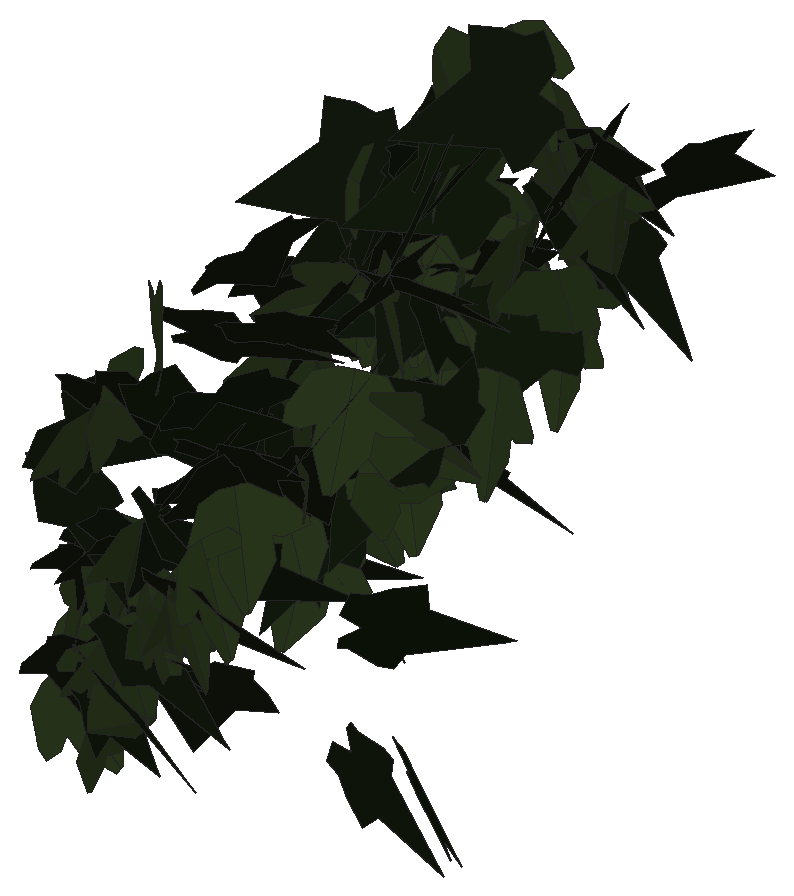
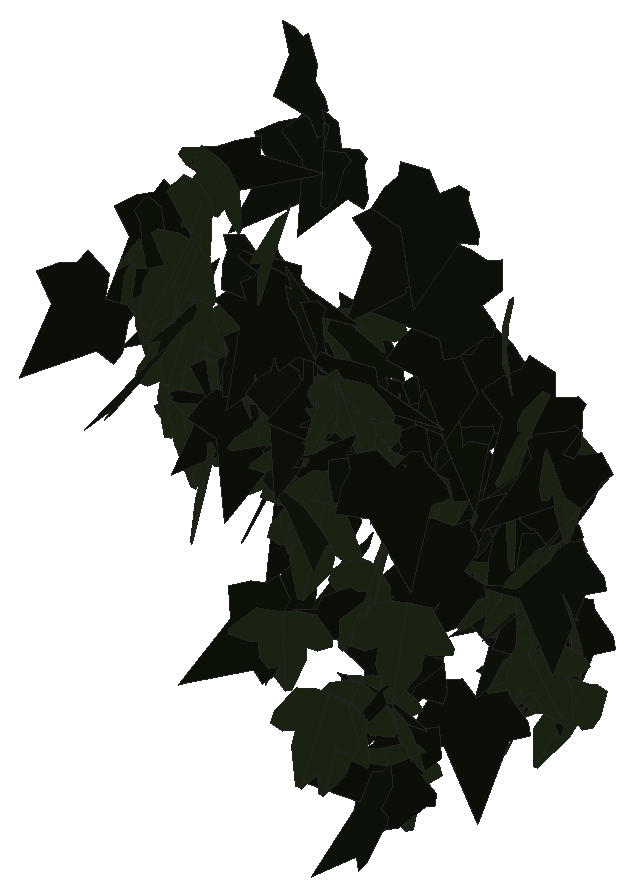
# SketchUp Ruby script. Lengths in inches.
U = 1.inch
M = Sketchup.active_model
def pt(a) = Geom::Point3d.new(a.map { |v| v * U })
def face(e, loops, mat)
  f = e.add_face(loops[0].map { |a| pt(a) })
  loops[1..].each { |l| e.add_face(l.map { |a| pt(a) }).erase! }
  f.material = f.back_material = mat if mat
  f
end
# faces: each face lists its corners as indices into pts; further lists are holes
def faces(e, pts, list, mat = nil) = list.each { |f| face(e, (f[0].is_a?(Array) ? f : [f]).map { |l| l.map { |i| pts[i] } }, mat) }
# xy, xz, yz: faces in a plane at the given z, y or x. An outline is a flat list of corners, or four numbers for a rectangle; further outlines are holes
def ring(l) = l.size == 4 ? [[l[0], l[1]], [l[2], l[1]], [l[2], l[3]], [l[0], l[3]]] : l.each_slice(2).to_a
def flat(e, list, mat, &to3) = list.each { |f| face(e, (f[0].is_a?(Array) ? f : [f]).map { |l| ring(l).map { |u, v| to3.(u, v) } }, mat) }
def xy(e, z, list, mat = nil) = flat(e, list, mat) { |x, y| [x, y, z] }
def xz(e, y, list, mat = nil) = flat(e, list, mat) { |x, z| [x, y, z] }
def yz(e, x, list, mat = nil) = flat(e, list, mat) { |y, z| [x, y, z] }
def lines(e, pts, list) = list.each { |a, b| e.add_line(pt(pts[a]), pt(pts[b])) }
# prism: a flat outline (further loops are holes) pulled along v
def prism(e, loops, v, mat = nil)
  f = face(e, loops, mat); d = Geom::Vector3d.new(v.map { |x| x * U })
  f.pushpull(f.normal.samedirection?(d) ? d.length : -d.length)
end
def box(e, o, s, mat = nil) = prism(e, [[o, [o[0] + s[0], o[1], o[2]], [o[0] + s[0], o[1] + s[1], o[2]], [o[0], o[1] + s[1], o[2]]]], [0, 0, s[2]], mat)
def at(x, y, z, deg = 0) = Geom::Transformation.translation(pt([x, y, z])) * Geom::Transformation.rotation(ORIGIN, Z_AXIS, deg.degrees)
def axes(o, x, y, z) = Geom::Transformation.new([*x, 0, *y, 0, *z, 0, *pt(o).to_a, 1])
def part(name) = M.definitions.add(name)
# library, detail: a bought-in or finely detailed component or shape, given as its bounding box
def library(name, o, s) = part(name).tap { |d| box(d.entities, o, s) }
def detail(e, o, s) = box(e.add_group.entities, o, s)
def put(e, d, t, mat = nil) = e.add_instance(d, t).tap { |i| i.material = mat if mat }
def group(e, t, mat = nil) = e.add_group.tap { |g| g.transformation = t; g.material = mat if mat }.entities
root = M.entities
M.materials.add("efeu1").color = [18, 25, 13]
M.materials.add("efeu2").color = [43, 57, 29]
c1 = part("ivyleaf_9")
p = [[1.54,2.16,1.25],[1.36,2.04,1.19],[-0.21,0.99,0.68],[-0.71,1.11,0.82],[-0.85,0.86,0.67],[-0.8,0.17,0.21],
  [-0.9,-0.01,0.1],[-0.67,-0.16,-0.02],[-0.08,-0.08,-0.05],[-0.03,-0.6,-0.4],[0.65,-0.88,-0.66],[0.83,-0.6,-0.49],
  [1.29,-0.42,-0.43],[1.8125,-0.07,-0.26],[1.21,0.44,0.15]]
faces(c1.entities,p,[[0,1,2,3,4,5,6,7,8,9,10,11,12,13,14]],"efeu1")
c2 = part("ivyleaf_10")
p = [[0,0.5,-0.03],[-0.0625,2.02,-0.43],[-0.19,2.01,-0.46],[-0.54,1.05,-0.29],[-0.52,0.625,-0.18],[-0.83,0.76,-0.28],
  [-1.16,0.64,-0.33],[-1.15,0.33,-0.24],[-0.77,-0.39,0.02],[-0.3,-0.51,0.16],[0.04,-0.48,0.23],[-0.02,2.01,-0.4375],
  [-0.06,2.01,-0.43],[0.04,-0.49,0.23],[0.67,-0.49,0.14],[1.38,0.36,-0.2],[1.375,0.51,-0.24],[0.81,0.65,-0.19],
  [0.62,0.59,-0.15],[0.6,1.09,-0.28],[0.5,1.23,-0.31]]
faces(c2.entities,p,[[0,1,2,3,4,5,6,7,8,9,10],[11,12,0,13,14,15,16,17,18,19,20]],"efeu2")
put(root,c1,axes([34.97,224.375,226.84],[0.18635,-0.03833,0.46239],[0.45579,-0.07806,-0.19016],[0.08677,0.49238,0.00585]))
put(root,c1,axes([33.65,224.56,225.77],[0.23627,-0.43906,-0.03737],[0.01842,0.05221,-0.49693],[0.44027,0.23344,0.04084]))
put(root,c1,axes([38.15,224.08,230.05],[0.09512,0.13668,0.47145],[0.01693,0.47903,-0.14229],[-0.49058,0.04304,0.08651]))
put(root,c2,axes([34.26,224.52,224.04],[-0.01331,-0.49982,-0.00062],[0.00269,0.00055,-0.49999],[0.49982,-0.01332,0.00267]))
put(root,c1,axes([36.35,224.14,228.54],[0.41156,0.27456,0.07234],[-0.00014,0.12759,-0.48345],[-0.28393,0.39792,0.1051]))
put(root,c2,axes([34.46,224.55,225.35],[0.05486,-0.49669,0.01713],[0.00671,-0.01649,-0.49968],[0.49694,0.05505,0.00486]))
put(root,c2,axes([33.9,224.47,226.4],[-0.0166,-0.49344,-0.07903],[0.00415,0.07893,-0.49371],[0.49971,-0.01705,0.00148]))
put(root,c2,axes([35.52,224.38,225.48],[0.07164,0.49096,0.06186],[0.00259,0.06213,-0.49612],[-0.49483,0.07141,0.00636]))
put(root,c1,axes([34.09,224.57,223.64],[0.35748,-0.3082,0.165],[0.14154,-0.0882,-0.47137],[0.31965,0.38372,0.02419]))
put(root,c1,axes([34.47,224.5,224.3125],[0.33175,-0.37154,-0.04357],[0.07631,0.12422,-0.47827],[0.36622,0.31069,0.13913]))
put(root,c1,axes([35.02,224.45,224.89],[0.39681,-0.14655,0.26658],[0.27236,-0.02402,-0.41862],[0.1355,0.47744,0.06077]))
put(root,c2,axes([35.15,224.43,225.04],[0.05746,-0.46499,-0.17458],[0.00556,0.17634,-0.46784],[0.49666,0.05183,0.02544]))
put(root,c2,axes([35.17,224.42,224.99],[-0.14905,0.47635,0.02964],[-0.00164,0.03054,-0.49906],[-0.47726,-0.14887,-0.00754]))
put(root,c1,axes([34.05,224.36,224.1],[0.19728,0.42233,-0.18089],[-0.08261,-0.16105,-0.46609],[-0.45195,0.21379,0.00624]))
put(root,c1,axes([36.08,224.24,229.21],[0.12055,0.48298,0.04692],[-0.00865,0.05048,-0.49737],[-0.48517,0.1191,0.02053]))
put(root,c1,axes([35.36,224.36,228.01],[0.38179,-0.06892,0.31542],[0.32286,0.08327,-0.3726],[-0.00117,0.48818,0.10809]))
put(root,c1,axes([34.23,224.31,227.04],[0.45045,0.21425,-0.03449],[-0.04369,0.0117,-0.49795],[-0.21257,0.45162,0.02926]))
put(root,c1,axes([37.56,224.28,225.56],[0.33918,0.12741,0.34457],[0.32373,0.11804,-0.36231],[-0.17367,0.46886,-0.00241]))
put(root,c1,axes([37.66,224.1875,229.3],[0.10481,0.41722,0.25484],[0.01741,0.25728,-0.42838],[-0.48858,0.09866,0.0394]))
put(root,c2,axes([34.25,224.24,223.32],[0.01123,-0.18738,-0.46343],[0.07848,0.45846,-0.18346],[0.49368,-0.06862,0.0397]))
put(root,c2,axes([33.71,224.64,224.45],[0.33781,-0.36812,-0.01926],[0.01049,0.03571,-0.49861],[0.36847,0.33647,0.03185]))
put(root,c2,axes([34.96,224.27,227.7],[-0.0367,0.04037,-0.49701],[-0.20273,0.4541,0.05186],[0.45558,0.20533,-0.01696]))
put(root,c1,axes([34.48,224.54,225.44],[0.19978,0.33296,-0.315],[-0.16852,-0.2662,-0.38825],[-0.42625,0.2613,0.00586]))
put(root,c2,axes([34.75,224.52,224.67],[-0.11062,0.487,0.02429],[-0.00816,0.02306,-0.4994],[-0.48754,-0.11089,0.00284]))
put(root,c2,axes([34.3,224.57,224.19],[-0.35728,-0.33193,-0.11033],[0.11029,0.04276,-0.48581],[0.33194,-0.37148,0.04266]))
put(root,c1,axes([34.68,224.66,225.64],[0.37166,-0.33425,-0.01217],[-0.01358,0.0031,-0.49981],[0.33419,0.37184,-0.00678]))
put(root,c1,axes([35.62,224.39,227.39],[0.23033,0.43977,-0.05959],[-0.02845,-0.05237,-0.49644],[-0.44287,0.23208,0.0009]))
put(root,c1,axes([35.55,224.43,226.69],[-0.08089,0.4934,0.00325],[-0.00346,0.00273,-0.49998],[-0.4934,-0.08091,0.00297]))
put(root,c1,axes([34.31,224.57,225.24],[-0.0586,0.4589,-0.18969],[-0.01655,-0.1927,-0.46108],[-0.49628,-0.04776,0.03778]))
put(root,c1,axes([33.99,224.54,223.71],[0.285,-0.246,-0.32903],[-0.24122,0.22395,-0.37638],[0.33255,0.37327,0.00897]))
put(root,c2,axes([34.86,224.47,224.7],[-0.11811,-0.34206,-0.34503],[0.13572,0.31771,-0.36144],[0.46651,-0.17903,0.0178]))
put(root,c2,axes([34.27,224.43,226.83],[0.01596,-0.28426,-0.41103],[0.11959,0.40146,-0.273],[0.48522,-0.0896,0.0808]))
put(root,c1,axes([35.58,224.45,226.71],[0.41641,0.25774,-0.10087],[-0.13834,0.03599,-0.47913],[-0.23972,0.42694,0.10129]))
put(root,c1,axes([37.11,224.65,223.79],[0.37319,-0.29128,-0.16089],[-0.08169,0.15415,-0.46858],[0.32258,0.37602,0.06747]))
put(root,c1,axes([35.2,224.42,226.07],[0.27285,0.01724,0.41864],[0.32924,0.30016,-0.22695],[-0.25914,0.39951,0.15244]))
put(root,c1,axes([37.75,224.47,229.36],[0.48326,0.12752,0.01403],[-0.02325,0.14081,-0.4792],[-0.12616,0.4625,0.14203]))
put(root,c1,axes([33.78,224.42,226.45],[0.05481,0.0184,-0.49665],[-0.08435,0.49275,0.00894],[0.48978,0.0828,0.05711]))
put(root,c2,axes([34.07,224.62,225],[-0.03441,0.48265,0.12597],[0.00493,0.1266,-0.48368],[-0.49879,-0.03205,-0.01347]))
put(root,c1,axes([34,224.6,225.05],[0.15996,0.45543,-0.13037],[-0.14225,-0.08507,-0.47173],[-0.45186,0.188,0.10235]))
put(root,c2,axes([35.54,224.79,225.89],[0.25289,0.43,0.03383],[0.01791,0.02871,-0.49885],[-0.43096,0.25352,-0.00088]))
put(root,c1,axes([34.22,224.55,223.96],[0.42873,0.25704,-0.01107],[-0.08616,0.12317,-0.47687],[-0.24243,0.4108,0.14991]))
put(root,c2,axes([33.5625,224.66,223.26],[0.14624,0.40594,0.25265],[0.06465,0.24499,-0.43105],[-0.47375,0.15874,0.01916]))
put(root,c2,axes([36.78,224.95,227.55],[0.42652,0.25364,-0.06118],[-0.05138,-0.0333,-0.49624],[-0.25581,0.4296,-0.00235]))
put(root,c1,axes([37.66,224.84,223.68],[0.37525,-0.06365,-0.32425],[-0.312,0.09333,-0.3794],[0.10882,0.48707,0.03033]))
put(root,c1,axes([36.74,224.74,227.32],[-0.07383,0.45234,0.19984],[-0.04646,0.19481,-0.45814],[-0.49233,-0.08622,0.01327]))
put(root,c2,axes([34.01,225.05,224.01],[-0.06553,0.4942,-0.03832],[0.02094,-0.03586,-0.49827],[-0.49525,-0.0669,-0.016]))
put(root,c2,axes([33.75,225.21,223.9],[0.36328,0.29795,-0.17103],[-0.14426,-0.09361,-0.4695],[-0.31179,0.39046,0.01795]))
put(root,c1,axes([36,224.92,226.5625],[0.32823,0.36541,-0.09349],[-0.09347,-0.04126,-0.48945],[-0.36541,0.33878,0.04122]))
put(root,c2,axes([37.13,225.11,227.23],[0.14676,-0.04549,0.47581],[0.43833,0.21128,-0.115],[-0.19059,0.45088,0.1019]))
put(root,c2,axes([36.1,225.09,226.32],[-0.01835,0.05933,-0.49613],[-0.18096,0.46197,0.06194],[0.46574,0.18183,0.00452]))
put(root,c1,axes([37.7,225.25,227.21],[-0.12889,0.31143,0.36933],[-0.26609,0.27327,-0.32329],[-0.40322,-0.27988,0.09529]))
put(root,c1,axes([34.93,225.24,224.82],[0.39504,0.11042,0.28592],[0.26654,0.1065,-0.40941],[-0.15132,0.47588,0.02528]))
put(root,c2,axes([36.79,225.4,226.52],[0.02656,-0.16915,-0.46977],[0.28001,0.39454,-0.12623],[0.41339,-0.25637,0.11569]))
put(root,c1,axes([34.36,225.625,223.33],[0.27028,0.33175,-0.25862],[-0.19766,-0.17119,-0.42617],[-0.37132,0.33261,0.03861]))
put(root,c2,axes([37.81,225.88,227.47],[0.48557,-0.08914,0.07925],[0.0791,-0.00798,-0.49364],[0.08927,0.49193,0.00635]))
put(root,c2,axes([36.29,226.39,226.1],[0.40949,0.27125,0.0935],[0.07274,0.05946,-0.49109],[-0.27754,0.4158,0.00923]))
put(root,c1,axes([37.48,226.91,230.26],[-0.31936,-0.17974,0.34015],[-0.29297,-0.17291,-0.36643],[0.24936,-0.43335,0.00513]))
put(root,c1,axes([36.78,226.96,229.04],[-0.43607,-0.04937,0.2396],[-0.24019,-0.00648,-0.43848],[0.0464,-0.49751,-0.01807]))
put(root,c2,axes([35.59,226.97,227.51],[-0.19592,0.22951,-0.39867],[0.23812,-0.32016,-0.30133],[-0.39359,-0.30793,0.01615]))
put(root,c2,axes([34.5,226.79,224.76],[0.30737,0.37801,0.11238],[0.06557,0.09151,-0.48716],[-0.38887,0.31422,0.00668]))
put(root,c2,axes([35.13,227.04,227.15],[0.13266,0.16472,-0.45307],[-0.45772,-0.10446,-0.172],[-0.15132,0.46038,0.12308]))
put(root,c1,axes([35.14,226.96,227.28],[-0.19985,0.39523,-0.23207],[0.0831,-0.21772,-0.44237],[-0.45073,-0.21539,0.02134]))
put(root,c1,axes([35.9,226.6875,226.38],[0.32872,0.37577,0.02711],[0.01844,0.01989,-0.49926],[-0.3763,0.32924,-0.00078]))
put(root,c1,axes([35.95,227.17,229.1875],[-0.38006,0.16701,-0.27868],[0.24981,-0.124,-0.41499],[-0.20773,-0.45468,0.01081]))
put(root,c1,axes([34.5,226.73,224.53],[0.24677,0.42688,0.08291],[0.03885,0.07331,-0.49307],[-0.43312,0.24979,0.00302]))
put(root,c1,axes([36.76,226.88,229.27],[-0.15033,0.47683,0.00594],[-0.00217,0.00555,-0.49996],[-0.47686,-0.15034,0.0004]))
put(root,c2,axes([37.1,227.25,230.47],[-0.39682,0.05542,-0.29911],[0.24243,-0.23935,-0.36598],[-0.18374,-0.43548,0.16308]))
put(root,c1,axes([35.36,227.22,228.21],[-0.46425,0.18541,0.00945],[-0.01291,-0.00686,-0.49979],[-0.18521,-0.4643,0.01115]))
put(root,c2,axes([35.49,227.34,226.63],[-0.01902,0.44977,-0.21759],[-0.01191,-0.21809,-0.44977],[-0.4995,-0.01193,0.01901]))
put(root,c1,axes([37.95,227.23,229.65],[-0.2531,0.38959,-0.18482],[0.11116,-0.14812,-0.46444],[-0.41664,-0.27619,-0.01163]))
put(root,c2,axes([36.96,227.35,228.26],[0.08534,-0.48994,0.05171],[0.00389,-0.05181,-0.49729],[0.49265,0.08528,-0.00503]))
put(root,c1,axes([35.15,227.38,228.39],[-0.42867,0.0275,0.25591],[-0.25587,0.00823,-0.42949],[-0.02783,-0.49918,0.00701]))
put(root,c1,axes([37.09,227.5,227.52],[-0.38831,-0.31472,-0.01277],[0.00587,0.01304,-0.4998],[0.31493,-0.3883,-0.00643]))
put(root,c2,axes([36.57,226.93,228.71],[0.03638,0.22719,0.44391],[0.02907,0.44337,-0.2293],[-0.49783,0.04249,0.01905]))
put(root,c2,axes([36.23,227.15,230],[-0.17319,0.45877,0.09765],[-0.03905,0.08963,-0.49035],[-0.46742,-0.17747,0.00478]))
put(root,c1,axes([35.59,227.61,227.51],[-0.15469,-0.46584,0.09523],[-0.00989,-0.09697,-0.49041],[0.47537,-0.1536,0.02079]))
put(root,c1,axes([34.4,227.17,227.23],[0.06342,0.46595,-0.1699],[-0.05182,-0.16412,-0.46945],[-0.49325,0.07715,0.02747]))
put(root,c2,axes([37.4,227.32,229.98],[-0.43378,0.22704,-0.10145],[0.0729,-0.07892,-0.48832],[-0.23775,-0.43844,0.03537]))
put(root,c1,axes([33.9,227.73,224.94],[0.01319,-0.3775,0.3276],[0.01468,-0.32728,-0.37772],[0.49961,0.01958,0.00245]))
put(root,c1,axes([35.36,227.76,227.11],[-0.26095,-0.25198,0.34411],[-0.19187,-0.29092,-0.35854],[0.3809,-0.31918,0.05513]))
put(root,c2,axes([34.67,227.35,225.63],[-0.45909,0.14851,-0.13109],[0.11944,-0.05645,-0.48223],[-0.15803,-0.47409,0.01635]))
put(root,c2,axes([34.95,227.4375,228.26],[0.49214,0.03381,-0.08156],[-0.08172,-0.00034,-0.49328],[-0.03341,0.49886,0.00519]))
put(root,c1,axes([35.55,227,227.6875],[0.08856,0.1353,0.47313],[0.14656,0.45166,-0.15659],[-0.46976,0.16641,0.04034]))
put(root,c1,axes([36.15,227.35,228.51],[0.02247,0.42737,-0.25855],[-0.13194,-0.24454,-0.41568],[-0.48175,0.08691,0.10178]))
put(root,c1,axes([35.13,227.71,225.3],[-0.28217,-0.41106,0.03757],[-0.01522,-0.03513,-0.49853],[0.41249,-0.28248,0.00731]))
put(root,c1,axes([34.4375,227.65,224.36],[-0.46353,-0.10897,-0.15253],[0.16173,-0.02675,-0.47236],[0.09479,-0.48725,0.06005]))
put(root,c2,axes([36.63,227.58,228.11],[0.37843,-0.26713,0.18823],[0.17947,-0.07078,-0.46128],[0.27309,0.41669,0.04231]))
put(root,c1,axes([36.02,227.2,229],[0.38929,0.31376,-0.00207],[-0.0002,-0.00305,-0.49999],[-0.31377,0.38928,-0.00225]))
put(root,c1,axes([37.32,227.49,228.74],[0.36138,-0.34555,0.00106],[0.03969,0.03999,-0.49682],[0.34326,0.35916,0.05633]))
put(root,c2,axes([35.64,227.5,227.64],[0.45072,0.20923,-0.05547],[-0.06001,-0.00232,-0.49638],[-0.20798,0.45411,0.02302]))
put(root,c2,axes([37.43,227.45,227.89],[-0.39815,-0.29215,-0.07825],[0.0674,0.04041,-0.49379],[0.29485,-0.40375,0.0072]))
put(root,c1,axes([37.68,227.32,229.57],[0.48663,0.11484,-0.00064],[0.00262,-0.01387,-0.4998],[-0.11481,0.48643,-0.0141]))
put(root,c2,axes([37.99,227.53,228.89],[-0.03917,-0.49648,-0.04442],[0.02643,0.04242,-0.4975],[0.49776,-0.04132,0.02292]))
put(root,c1,axes([35.8,227.41,227.27],[0.33458,-0.24231,-0.28168],[-0.22638,0.16763,-0.4131],[0.29464,0.40396,0.00246]))
put(root,c1,axes([33.93,227.68,224.66],[0.07543,-0.4857,-0.09168],[-0.02724,0.08852,-0.49135],[0.49353,0.07912,-0.01311]))
put(root,c2,axes([33.92,227.66,224.13],[0.4022,-0.26395,0.13626],[0.12275,-0.06117,-0.48082],[0.2705,0.42022,0.01559]))
put(root,c2,axes([34.375,227.61,224.375],[0.46914,-0.02602,-0.17096],[-0.17084,0.0069,-0.46986],[0.02681,0.49927,-0.00241]))
put(root,c2,axes([37.32,227.43,229.47],[-0.23225,0.43595,0.07752],[-0.02543,0.07426,-0.4938],[-0.44206,-0.23331,-0.01232]))
put(root,c2,axes([36.33,227.31,227.76],[0.19314,-0.15284,0.43513],[-0.31354,0.30244,0.2454],[-0.33822,-0.36765,0.02098]))
put(root,c2,axes([36.33,227.57,227.76],[0.38568,0.31734,0.02346],[0.01956,0.01315,-0.49944],[-0.3176,0.38617,-0.00228]))
put(root,c2,axes([37.71,227.52,229.17],[-0.49277,-0.07941,-0.02949],[0.02754,0.01444,-0.49903],[0.08011,-0.49344,-0.00985]))
put(root,c2,axes([35.1,227.32,228.21],[-0.06084,0.35365,0.34818],[-0.08777,0.33759,-0.35823],[-0.48846,-0.10471,0.021]))
put(root,c2,axes([34.34,227.51,226.17],[-0.27068,0.40987,0.09351],[-0.06164,0.07132,-0.49103],[-0.41585,-0.27735,0.01192]))
put(root,c2,axes([35.86,227.56,227.35],[-0.24931,-0.33423,-0.27593],[0.29436,0.10307,-0.3908],[0.31812,-0.35731,0.14537]))
put(root,c2,axes([37.32,227.59,228.67],[-0.49651,0.0445,-0.03875],[0.03836,-0.00614,-0.49849],[-0.04484,-0.49798,0.00268]))
put(root,c2,axes([35.38,227.625,227.33],[0.34718,0.35669,0.04728],[0.03394,0.03295,-0.49776],[-0.35821,0.34884,-0.00134]))
put(root,c2,axes([37.44,227.59,229.375],[-0.47335,-0.05299,-0.1521],[0.15009,0.02616,-0.47622],[0.05843,-0.4965,-0.00886]))
put(root,c2,axes([35.3,227.53,226.89],[0.18941,0.43324,0.16258],[0.06076,0.15087,-0.47281],[-0.45873,0.19886,0.0045]))
put(root,c1,axes([36.34,227.39,227.78],[0.40447,0.26645,0.12414],[0.09607,0.07974,-0.48416],[-0.2778,0.41551,0.0133]))
put(root,c2,axes([37.13,227.78,227.1875],[0.48351,-0.07346,0.10404],[0.10311,-0.01396,-0.48905],[0.07476,0.49438,0.00165]))
put(root,c2,axes([35.2,227.6875,226.48],[-0.49243,-0.08134,-0.02995],[0.03139,-0.00626,-0.49897],[0.0808,-0.4933,0.01127]))
put(root,c2,axes([34.01,227.75,223.57],[0.41305,0.2679,-0.08726],[-0.1034,0.00009,-0.48919],[-0.2621,0.42217,0.05548]))
put(root,c2,axes([33.86,227.7,225.54],[-0.45272,-0.21135,-0.01952],[0.01581,0.01228,-0.4996],[0.21166,-0.45297,-0.00444]))
put(root,c1,axes([35.62,227.4375,227.97],[0.05928,0.46729,0.16772],[0.01593,0.16704,-0.471],[-0.49622,0.06118,0.00492]))
put(root,c1,axes([36.22,227.57,227.64],[0.19144,0.46115,0.02634],[-0.00959,0.03247,-0.49885],[-0.4618,0.1905,0.02128]))
put(root,c1,axes([33.66,227.67,223.49],[0.36963,-0.01655,0.3363],[0.33286,0.09324,-0.36127],[-0.05076,0.49095,0.07994]))
put(root,c1,axes([35.46,227.66,226.67],[-0.04624,0.38107,0.32039],[-0.16839,0.29083,-0.37022],[-0.46852,-0.14214,0.10144]))
put(root,c2,axes([34.42,227.99,224.37],[-0.27386,-0.36809,-0.19876],[0.19742,0.09573,-0.44929],[0.36882,-0.32457,0.0929]))
put(root,c1,axes([35.53,228.125,225.14],[0.49373,-0.05044,0.06072],[0.066,0.05287,-0.4928],[0.0433,0.49463,0.05887]))
put(root,c1,axes([37.37,228.33,228.11],[0.29376,-0.3917,-0.10138],[-0.01038,0.11794,-0.48578],[0.40447,0.28751,0.06117]))
put(root,c2,axes([36.42,228.33,227.11],[-0.31343,0.3853,0.05751],[-0.05097,0.03262,-0.49632],[-0.38622,-0.31698,0.01883]))
put(root,c1,axes([33.625,228.47,223.33],[0.43215,-0.24905,-0.03492],[-0.03714,0.00547,-0.49859],[0.24873,0.43353,-0.01377]))
put(root,c2,axes([35.06,228.5,225.45],[0.43238,0.25044,0.01802],[0.00884,0.02067,-0.49949],[-0.25093,0.43226,0.01345]))
put(root,c2,axes([34.17,228.49,224.4],[-0.48474,0.11583,-0.0401],[0.03688,-0.01817,-0.49831],[-0.11689,-0.48606,0.00907]))
put(root,c2,axes([34.43,228.58,224.47],[-0.49408,-0.04251,-0.06382],[0.0642,-0.00171,-0.49586],[0.04194,-0.49819,0.00715]))
put(root,c1,axes([38.01,228.4,228.91],[0.268,0.34588,0.24195],[0.12633,0.20774,-0.4369],[-0.40276,0.29531,0.02396]))
